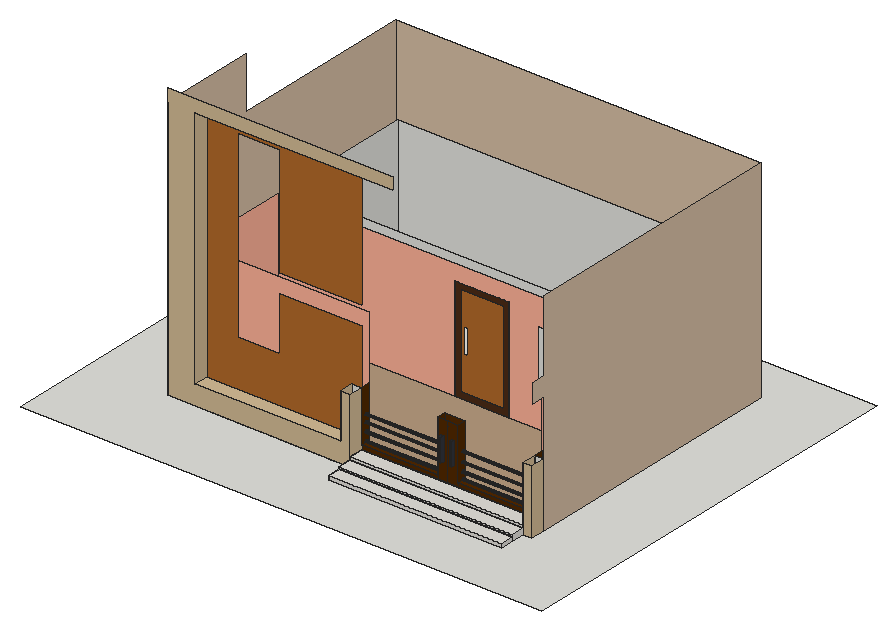
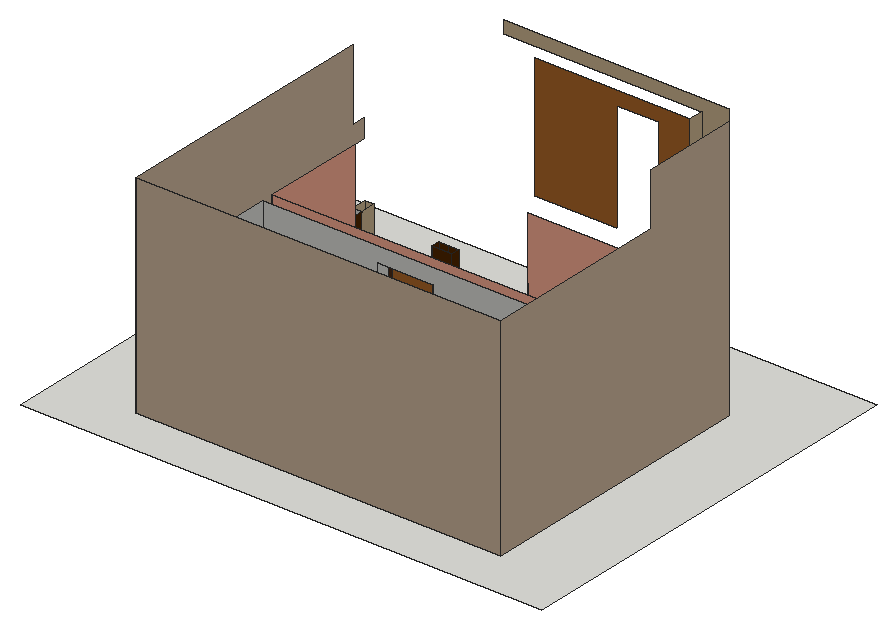
# SketchUp Ruby script. Lengths in inches.
U = 1.inch
M = Sketchup.active_model
def pt(a) = Geom::Point3d.new(a.map { |v| v * U })
def face(e, loops, mat)
  f = e.add_face(loops[0].map { |a| pt(a) })
  loops[1..].each { |l| e.add_face(l.map { |a| pt(a) }).erase! }
  f.material = f.back_material = mat if mat
  f
end
# faces: each face lists its corners as indices into pts; further lists are holes
def faces(e, pts, list, mat = nil) = list.each { |f| face(e, (f[0].is_a?(Array) ? f : [f]).map { |l| l.map { |i| pts[i] } }, mat) }
# xy, xz, yz: faces in a plane at the given z, y or x. An outline is a flat list of corners, or four numbers for a rectangle; further outlines are holes
def ring(l) = l.size == 4 ? [[l[0], l[1]], [l[2], l[1]], [l[2], l[3]], [l[0], l[3]]] : l.each_slice(2).to_a
def flat(e, list, mat, &to3) = list.each { |f| face(e, (f[0].is_a?(Array) ? f : [f]).map { |l| ring(l).map { |u, v| to3.(u, v) } }, mat) }
def xy(e, z, list, mat = nil) = flat(e, list, mat) { |x, y| [x, y, z] }
def xz(e, y, list, mat = nil) = flat(e, list, mat) { |x, z| [x, y, z] }
def yz(e, x, list, mat = nil) = flat(e, list, mat) { |y, z| [x, y, z] }
def lines(e, pts, list) = list.each { |a, b| e.add_line(pt(pts[a]), pt(pts[b])) }
# prism: a flat outline (further loops are holes) pulled along v
def prism(e, loops, v, mat = nil)
  f = face(e, loops, mat); d = Geom::Vector3d.new(v.map { |x| x * U })
  f.pushpull(f.normal.samedirection?(d) ? d.length : -d.length)
end
def box(e, o, s, mat = nil) = prism(e, [[o, [o[0] + s[0], o[1], o[2]], [o[0] + s[0], o[1] + s[1], o[2]], [o[0], o[1] + s[1], o[2]]]], [0, 0, s[2]], mat)
def at(x, y, z, deg = 0) = Geom::Transformation.translation(pt([x, y, z])) * Geom::Transformation.rotation(ORIGIN, Z_AXIS, deg.degrees)
def axes(o, x, y, z) = Geom::Transformation.new([*x, 0, *y, 0, *z, 0, *pt(o).to_a, 1])
def part(name) = M.definitions.add(name)
# library, detail: a bought-in or finely detailed component or shape, given as its bounding box
def library(name, o, s) = part(name).tap { |d| box(d.entities, o, s) }
def detail(e, o, s) = box(e.add_group.entities, o, s)
def put(e, d, t, mat = nil) = e.add_instance(d, t).tap { |i| i.material = mat if mat }
def group(e, t, mat = nil) = e.add_group.tap { |g| g.transformation = t; g.material = mat if mat }.entities
root = M.entities
M.materials.add("[Carpet Pattern Leaf Squares Tan]").color = [181, 154, 125]
M.materials.add("[Color B02]").color = [255, 178, 153]
M.materials.add("[Color C07]").color = [81, 40, 0]
M.materials.add("[Formica Beige]").color = [211, 187, 149]
M.materials.add("[Formica Laminate Dark]").color = [50, 53, 60]
M.materials.add("[Formica Laminate Light]").color = [213, 189, 164]
M.materials.add("[Marble Carrara Gold Floor Tile]").color = [225, 223, 217]
M.materials.add("[Wood Bamboo]").color = [177, 105, 43]
M.materials.add("[Wood Veneer 01]").color = [76, 44, 23]
xy(root,0,[[[0,0,523.75,420.4375],[262.04,59.3,436.45,59.3,436.45,86.05,445.45,86.05,445.45,373.42,79.02,373.42,79.02,86.05,262.04,86.05]],[262.04,59.3,436.45,72.67],[262.04,72.67,436.45,86.05],[79.02,86.05,79.02,373.42,445.45,373.42,445.45,100.8,246.1,100.8,246.1,86.05],[246.1,86.05,262.24,100.8],
  [262.24,86.05,436.45,100.8],[436.45,86.05,445.45,100.8]])
xy(root,3.75,[[262.04,59.3,436.45,72.67]],"[Marble Carrara Gold Floor Tile]")
xy(root,6.125,[[262.04,72.67,436.45,86.05]],"[Marble Carrara Gold Floor Tile]")
xy(root,9,[[266,213.0625,320.78,224.66],[88.02,224.66,436.45,364.42]])
xy(root,9,[[88.02,109.8,436.45,213.0625]],"[Carpet Pattern Leaf Squares Tan]")
xy(root,9,[[262.24,86.05,436.45,100.8]],"[Marble Carrara Gold Floor Tile]")
xy(root,13.11,[[359.13,106.01,436.45,109.8]])
xy(root,13.11,[[262.24,100.8,338.39,109.8],[359.13,100.8,436.45,106.01]],"[Color C07]")
xy(root,19.9,[[106.35,86.05,252.91,100.8]],"[Formica Beige]")
xy(root,27.09,[[342.13,97.98,344.57,100.8],[352.82,97.98,355.26,100.8]],"[Formica Laminate Dark]")
xz(root,59.3,[[262.04,0,436.45,3.75]],"[Marble Carrara Gold Floor Tile]")
xz(root,72.67,[[262.04,0,436.45,3.75]])
xz(root,72.67,[[262.04,3.75,436.45,6.125]],"[Marble Carrara Gold Floor Tile]")
xz(root,86.05,[[262.04,0,262.24,6.125],[262.24,0,436.45,6.125],[262.04,6.125,262.24,64.77]])
xz(root,86.05,[[79.02,0,262.04,0,262.04,64.77,252.91,64.77,252.91,19.9,106.35,19.9,106.35,264.08,305.61,264.08,305.61,276.4375,79.02,276.4375],[436.45,0,445.45,64.77]],"[Formica Beige]")
xz(root,86.05,[[262.24,6.125,436.45,9]],"[Marble Carrara Gold Floor Tile]")
xz(root,97.98,[[342.13,27.09,344.57,49.9],[352.82,27.09,355.26,49.9]],"[Formica Laminate Dark]")
xz(root,100.8,[[246.1,0,262.24,0,262.24,64.77,252.91,64.77,252.91,19.9,246.1,19.9],[262.24,0,338.39,9],[338.39,0,348.76,9],[348.76,0,359.13,9],[359.13,0,436.45,9],
  [436.45,0,445.45,64.77]])
xz(root,100.8,[[262.24,9,338.39,13.11],[[338.39,9,348.76,64.77],[342.13,27.09,344.57,49.9]],[[348.76,9,359.13,64.77],[352.82,27.09,355.26,49.9]],[359.13,9,436.45,13.11]],"[Color C07]")
xz(root,100.8,[[106.35,19.9,252.91,19.9,252.91,64.77,262.24,64.77,262.24,120.54,180.23,120.54,180.23,66.71,137.86,66.71,137.86,250,180.23,250,180.23,139.625,262.24,139.625,262.24,264.08,106.35,264.08]],"[Wood Bamboo]")
xz(root,109.8,[[262.24,9,338.39,13.11],[359.13,9,436.45,13.11]])
xz(root,109.8,[[88.02,9,262.24,129]],"[Color B02]")
xz(root,109.8,[[338.39,9,359.13,64.77]],"[Color C07]")
xz(root,213.0625,[[[88.02,9,266,9,266,113.3,320.78,113.3,320.78,9,436.45,9,436.45,129,88.02,129],[349.875,43.38,418,101.95]]],"[Color B02]")
xz(root,213.0625,[[[271.87,14.87,314.91,107.4375],[275.21,50.38,279.02,74.76]]],"[Wood Bamboo]")
xz(root,213.0625,[[[266,9,320.78,113.3],[271.87,14.87,314.91,107.4375]]],"[Wood Veneer 01]")
xz(root,224.66,[[[88.02,9,88.02,129,436.45,129,436.45,9,320.78,9,320.78,113.3,266,113.3,266,9],[349.875,43.38,418,101.95]]])
xz(root,364.42,[[88.02,9,436.45,129]])
xz(root,373.42,[[79.02,0,445.45,211.625]],"[Formica Laminate Light]")
yz(root,79.02,[[86.05,0,86.05,264.08,184.36,264.08,184.36,211.625,373.42,211.625,373.42,0]],"[Formica Laminate Light]")
yz(root,88.02,[[224.66,9,364.42,129]])
yz(root,88.02,[[109.8,9,213.0625,129]],"[Color B02]")
yz(root,106.35,[[86.05,19.9,100.8,264.08]],"[Formica Beige]")
yz(root,252.91,[[86.05,19.9,100.8,64.77]],"[Formica Beige]")
yz(root,262.04,[[59.3,0,72.67,3.75],[72.67,0,86.05,6.125]],"[Marble Carrara Gold Floor Tile]")
yz(root,262.24,[[86.05,0,100.8,9],[105.68,13.86,105.43,13.9,105.18,14,104.98,14.15,104.82,14.36,104.72,14.6,104.68,14.86,104.72,15.12,104.82,15.36,104.98,15.57,105.18,15.73,105.43,15.83,105.68,15.86,105.94,15.83,106.18,15.73,106.39,15.57,106.55,15.36,106.65,15.12,106.68,14.86,106.65,14.6,106.55,14.36,106.39,14.15,106.18,14,105.94,13.9],[105.68,22.36,105.43,22.4,105.18,22.5,104.98,22.65,104.82,22.86,104.72,23.1,104.68,23.36,104.72,23.62,104.82,23.86,104.98,24.07,105.18,24.23,105.43,24.33,105.68,24.36,105.94,24.33,106.18,24.23,106.39,24.07,106.55,23.86,106.65,23.62,106.68,23.36,106.65,23.1,106.55,22.86,106.39,22.65,106.18,22.5,105.94,22.4],[105.68,30.61,105.43,30.65,105.18,30.75,104.98,30.9,104.82,31.11,104.72,31.35,104.68,31.61,104.72,31.87,104.82,32.11,104.98,32.32,105.18,32.48,105.43,32.58,105.68,32.61,105.94,32.58,106.18,32.48,106.39,32.32,106.55,32.11,106.65,31.87,106.68,31.61,106.65,31.35,106.55,31.11,106.39,30.9,106.18,30.75,105.94,30.65],[105.68,38.11,105.43,38.15,105.18,38.25,104.98,38.4,104.82,38.61,104.72,38.85,104.68,39.11,104.72,39.37,104.82,39.61,104.98,39.82,105.18,39.98,105.43,40.08,105.68,40.11,105.94,40.08,106.18,39.98,106.39,39.82,106.55,39.61,106.65,39.37,106.68,39.11,106.65,38.85,106.55,38.61,106.39,38.4,106.18,38.25,105.94,38.15]])
yz(root,262.24,[[[100.8,13.11,109.8,64.77],[105.68,13.86,105.43,13.9,105.18,14,104.98,14.15,104.82,14.36,104.72,14.6,104.68,14.86,104.72,15.12,104.82,15.36,104.98,15.57,105.18,15.73,105.43,15.83,105.68,15.86,105.94,15.83,106.18,15.73,106.39,15.57,106.55,15.36,106.65,15.12,106.68,14.86,106.65,14.6,106.55,14.36,106.39,14.15,106.18,14,105.94,13.9],[105.68,53.61,105.43,53.65,105.18,53.75,104.98,53.9,104.82,54.11,104.72,54.35,104.68,54.61,104.72,54.87,104.82,55.11,104.98,55.32,105.18,55.48,105.43,55.58,105.68,55.61,105.94,55.58,106.18,55.48,106.39,55.32,106.55,55.11,106.65,54.87,106.68,54.61,106.65,54.35,106.55,54.11,106.39,53.9,106.18,53.75,105.94,53.65],[105.68,22.36,105.43,22.4,105.18,22.5,104.98,22.65,104.82,22.86,104.72,23.1,104.68,23.36,104.72,23.62,104.82,23.86,104.98,24.07,105.18,24.23,105.43,24.33,105.68,24.36,105.94,24.33,106.18,24.23,106.39,24.07,106.55,23.86,106.65,23.62,106.68,23.36,106.65,23.1,106.55,22.86,106.39,22.65,106.18,22.5,105.94,22.4],[105.68,45.42,105.43,45.46,105.18,45.56,104.98,45.72,104.82,45.92,104.72,46.17,104.68,46.42,104.72,46.68,104.82,46.92,104.98,47.13,105.18,47.29,105.43,47.39,105.68,47.42,105.94,47.39,106.18,47.29,106.39,47.13,106.55,46.92,106.65,46.68,106.68,46.42,106.65,46.17,106.55,45.92,106.39,45.72,106.18,45.56,105.94,45.46],[105.68,30.61,105.43,30.65,105.18,30.75,104.98,30.9,104.82,31.11,104.72,31.35,104.68,31.61,104.72,31.87,104.82,32.11,104.98,32.32,105.18,32.48,105.43,32.58,105.68,32.61,105.94,32.58,106.18,32.48,106.39,32.32,106.55,32.11,106.65,31.87,106.68,31.61,106.65,31.35,106.55,31.11,106.39,30.9,106.18,30.75,105.94,30.65],[105.68,38.11,105.43,38.15,105.18,38.25,104.98,38.4,104.82,38.61,104.72,38.85,104.68,39.11,104.72,39.37,104.82,39.61,104.98,39.82,105.18,39.98,105.43,40.08,105.68,40.11,105.94,40.08,106.18,39.98,106.39,39.82,106.55,39.61,106.65,39.37,106.68,39.11,106.65,38.85,106.55,38.61,106.39,38.4,106.18,38.25,105.94,38.15],[105.68,60.05,105.43,60.08,105.18,60.18,104.98,60.34,104.82,60.55,104.72,60.79,104.68,61.05,104.72,61.31,104.82,61.55,104.98,61.76,105.18,61.92,105.43,62.02,105.68,62.05,105.94,62.02,106.18,61.92,106.39,61.76,106.55,61.55,106.65,61.31,106.68,61.05,106.65,60.79,106.55,60.55,106.39,60.34,106.18,60.18,105.94,60.08]]],"[Color C07]")
yz(root,262.24,[[86.05,9,100.8,64.77]],"[Formica Beige]")
yz(root,266,[[213.0625,9,224.66,113.3]])
yz(root,320.78,[[213.0625,9,224.66,113.3]])
yz(root,338.39,[[[100.8,13.11,109.8,64.77],[105.68,60.05,105.94,60.08,106.18,60.18,106.39,60.34,106.55,60.55,106.65,60.79,106.68,61.05,106.65,61.31,106.55,61.55,106.39,61.76,106.18,61.92,105.94,62.02,105.68,62.05,105.43,62.02,105.18,61.92,104.98,61.76,104.82,61.55,104.72,61.31,104.68,61.05,104.72,60.79,104.82,60.55,104.98,60.34,105.18,60.18,105.43,60.08],[105.68,53.61,105.94,53.65,106.18,53.75,106.39,53.9,106.55,54.11,106.65,54.35,106.68,54.61,106.65,54.87,106.55,55.11,106.39,55.32,106.18,55.48,105.94,55.58,105.68,55.61,105.43,55.58,105.18,55.48,104.98,55.32,104.82,55.11,104.72,54.87,104.68,54.61,104.72,54.35,104.82,54.11,104.98,53.9,105.18,53.75,105.43,53.65],[105.68,45.42,105.94,45.46,106.18,45.56,106.39,45.72,106.55,45.92,106.65,46.17,106.68,46.42,106.65,46.68,106.55,46.92,106.39,47.13,106.18,47.29,105.94,47.39,105.68,47.42,105.43,47.39,105.18,47.29,104.98,47.13,104.82,46.92,104.72,46.68,104.68,46.42,104.72,46.17,104.82,45.92,104.98,45.72,105.18,45.56,105.43,45.46],[105.68,38.11,105.94,38.15,106.18,38.25,106.39,38.4,106.55,38.61,106.65,38.85,106.68,39.11,106.65,39.37,106.55,39.61,106.39,39.82,106.18,39.98,105.94,40.08,105.68,40.11,105.43,40.08,105.18,39.98,104.98,39.82,104.82,39.61,104.72,39.37,104.68,39.11,104.72,38.85,104.82,38.61,104.98,38.4,105.18,38.25,105.43,38.15],[105.68,30.61,105.94,30.65,106.18,30.75,106.39,30.9,106.55,31.11,106.65,31.35,106.68,31.61,106.65,31.87,106.55,32.11,106.39,32.32,106.18,32.48,105.94,32.58,105.68,32.61,105.43,32.58,105.18,32.48,104.98,32.32,104.82,32.11,104.72,31.87,104.68,31.61,104.72,31.35,104.82,31.11,104.98,30.9,105.18,30.75,105.43,30.65],[105.68,22.36,105.94,22.4,106.18,22.5,106.39,22.65,106.55,22.86,106.65,23.1,106.68,23.36,106.65,23.62,106.55,23.86,106.39,24.07,106.18,24.23,105.94,24.33,105.68,24.36,105.43,24.33,105.18,24.23,104.98,24.07,104.82,23.86,104.72,23.62,104.68,23.36,104.72,23.1,104.82,22.86,104.98,22.65,105.18,22.5,105.43,22.4],[105.68,13.86,105.94,13.9,106.18,14,106.39,14.15,106.55,14.36,106.65,14.6,106.68,14.86,106.65,15.12,106.55,15.36,106.39,15.57,106.18,15.73,105.94,15.83,105.68,15.86,105.43,15.83,105.18,15.73,104.98,15.57,104.82,15.36,104.72,15.12,104.68,14.86,104.72,14.6,104.82,14.36,104.98,14.15,105.18,14,105.43,13.9]]],"[Color C07]")
yz(root,342.13,[[97.98,27.09,100.8,49.9]],"[Formica Laminate Dark]")
yz(root,344.57,[[97.98,27.09,100.8,49.9]],"[Formica Laminate Dark]")
yz(root,352.82,[[97.98,27.09,100.8,49.9]],"[Formica Laminate Dark]")
yz(root,355.26,[[97.98,27.09,100.8,49.9]],"[Formica Laminate Dark]")
yz(root,359.13,[[[100.8,13.11,109.8,64.77],[106.01,60.17,105.75,60.2,105.51,60.3,105.3,60.46,105.14,60.67,105.04,60.91,105.01,61.17,105.04,61.43,105.14,61.67,105.3,61.875,105.51,62.03,105.75,62.13,106.01,62.17,106.27,62.13,106.51,62.03,106.72,61.875,106.875,61.67,106.98,61.43,107.01,61.17,106.98,60.91,106.875,60.67,106.72,60.46,106.51,60.3,106.27,60.2],[106.01,53.17,105.75,53.2,105.51,53.3,105.3,53.46,105.14,53.67,105.04,53.91,105.01,54.17,105.04,54.43,105.14,54.67,105.3,54.875,105.51,55.03,105.75,55.13,106.01,55.17,106.27,55.13,106.51,55.03,106.72,54.875,106.875,54.67,106.98,54.43,107.01,54.17,106.98,53.91,106.875,53.67,106.72,53.46,106.51,53.3,106.27,53.2],[106.01,46.23,105.75,46.26,105.51,46.36,105.3,46.52,105.14,46.73,105.04,46.97,105.01,47.23,105.04,47.49,105.14,47.73,105.3,47.9375,105.51,48.1,105.75,48.2,106.01,48.23,106.27,48.2,106.51,48.1,106.72,47.9375,106.875,47.73,106.98,47.49,107.01,47.23,106.98,46.97,106.875,46.73,106.72,46.52,106.51,46.36,106.27,46.26],[106.01,38.36,105.75,38.39,105.51,38.49,105.3,38.65,105.14,38.86,105.04,39.1,105.01,39.36,105.04,39.61,105.14,39.86,105.3,40.0625,105.51,40.22,105.75,40.32,106.01,40.36,106.27,40.32,106.51,40.22,106.72,40.0625,106.875,39.86,106.98,39.61,107.01,39.36,106.98,39.1,106.875,38.86,106.72,38.65,106.51,38.49,106.27,38.39],[106.01,28.73,105.75,28.76,105.51,28.86,105.3,29.02,105.14,29.23,105.04,29.47,105.01,29.73,105.04,29.99,105.14,30.23,105.3,30.4375,105.51,30.6,105.75,30.7,106.01,30.73,106.27,30.7,106.51,30.6,106.72,30.4375,106.875,30.23,106.98,29.99,107.01,29.73,106.98,29.47,106.875,29.23,106.72,29.02,106.51,28.86,106.27,28.76],[106.01,19.98,105.75,20.01,105.51,20.11,105.3,20.27,105.14,20.48,105.04,20.72,105.01,20.98,105.04,21.24,105.14,21.48,105.3,21.6875,105.51,21.85,105.75,21.95,106.01,21.98,106.27,21.95,106.51,21.85,106.72,21.6875,106.875,21.48,106.98,21.24,107.01,20.98,106.98,20.72,106.875,20.48,106.72,20.27,106.51,20.11,106.27,20.01],[106.01,13.11,105.75,13.14,105.51,13.24,105.3,13.4,105.14,13.61,105.04,13.85,105.01,14.11,105.04,14.36,105.14,14.61,105.3,14.8125,105.51,14.97,105.75,15.07,106.01,15.11,106.27,15.07,106.51,14.97,106.72,14.8125,106.875,14.61,106.98,14.36,107.01,14.11,106.98,13.85,106.875,13.61,106.72,13.4,106.51,13.24,106.27,13.14]]],"[Color C07]")
yz(root,436.45,[[86.05,0,100.8,9],[224.66,9,364.42,129],[106.01,13.11,106.27,13.14,106.51,13.24,106.72,13.4,106.875,13.61,106.98,13.85,107.01,14.11,106.98,14.36,106.875,14.61,106.72,14.8125,106.51,14.97,106.27,15.07,106.01,15.11,105.75,15.07,105.51,14.97,105.3,14.8125,105.14,14.61,105.04,14.36,105.01,14.11,105.04,13.85,105.14,13.61,105.3,13.4,105.51,13.24,105.75,13.14],[106.01,19.98,106.27,20.01,106.51,20.11,106.72,20.27,106.875,20.48,106.98,20.72,107.01,20.98,106.98,21.24,106.875,21.48,106.72,21.6875,106.51,21.85,106.27,21.95,106.01,21.98,105.75,21.95,105.51,21.85,105.3,21.6875,105.14,21.48,105.04,21.24,105.01,20.98,105.04,20.72,105.14,20.48,105.3,20.27,105.51,20.11,105.75,20.01],[106.01,28.73,106.27,28.76,106.51,28.86,106.72,29.02,106.875,29.23,106.98,29.47,107.01,29.73,106.98,29.99,106.875,30.23,106.72,30.4375,106.51,30.6,106.27,30.7,106.01,30.73,105.75,30.7,105.51,30.6,105.3,30.4375,105.14,30.23,105.04,29.99,105.01,29.73,105.04,29.47,105.14,29.23,105.3,29.02,105.51,28.86,105.75,28.76],
  [106.01,38.36,106.27,38.39,106.51,38.49,106.72,38.65,106.875,38.86,106.98,39.1,107.01,39.36,106.98,39.61,106.875,39.86,106.72,40.0625,106.51,40.22,106.27,40.32,106.01,40.36,105.75,40.32,105.51,40.22,105.3,40.0625,105.14,39.86,105.04,39.61,105.01,39.36,105.04,39.1,105.14,38.86,105.3,38.65,105.51,38.49,105.75,38.39]])
yz(root,436.45,[[109.8,9,213.0625,129]],"[Color B02]")
yz(root,436.45,[[[100.8,13.11,109.8,64.77],[106.01,13.11,106.27,13.14,106.51,13.24,106.72,13.4,106.875,13.61,106.98,13.85,107.01,14.11,106.98,14.36,106.875,14.61,106.72,14.8125,106.51,14.97,106.27,15.07,106.01,15.11,105.75,15.07,105.51,14.97,105.3,14.8125,105.14,14.61,105.04,14.36,105.01,14.11,105.04,13.85,105.14,13.61,105.3,13.4,105.51,13.24,105.75,13.14],[106.01,53.17,106.27,53.2,106.51,53.3,106.72,53.46,106.875,53.67,106.98,53.91,107.01,54.17,106.98,54.43,106.875,54.67,106.72,54.875,106.51,55.03,106.27,55.13,106.01,55.17,105.75,55.13,105.51,55.03,105.3,54.875,105.14,54.67,105.04,54.43,105.01,54.17,105.04,53.91,105.14,53.67,105.3,53.46,105.51,53.3,105.75,53.2],[106.01,19.98,106.27,20.01,106.51,20.11,106.72,20.27,106.875,20.48,106.98,20.72,107.01,20.98,106.98,21.24,106.875,21.48,106.72,21.6875,106.51,21.85,106.27,21.95,106.01,21.98,105.75,21.95,105.51,21.85,105.3,21.6875,105.14,21.48,105.04,21.24,105.01,20.98,105.04,20.72,105.14,20.48,105.3,20.27,105.51,20.11,105.75,20.01],[106.01,46.23,106.27,46.26,106.51,46.36,106.72,46.52,106.875,46.73,106.98,46.97,107.01,47.23,106.98,47.49,106.875,47.73,106.72,47.9375,106.51,48.1,106.27,48.2,106.01,48.23,105.75,48.2,105.51,48.1,105.3,47.9375,105.14,47.73,105.04,47.49,105.01,47.23,105.04,46.97,105.14,46.73,105.3,46.52,105.51,46.36,105.75,46.26],[106.01,28.73,106.27,28.76,106.51,28.86,106.72,29.02,106.875,29.23,106.98,29.47,107.01,29.73,106.98,29.99,106.875,30.23,106.72,30.4375,106.51,30.6,106.27,30.7,106.01,30.73,105.75,30.7,105.51,30.6,105.3,30.4375,105.14,30.23,105.04,29.99,105.01,29.73,105.04,29.47,105.14,29.23,105.3,29.02,105.51,28.86,105.75,28.76],[106.01,38.36,106.27,38.39,106.51,38.49,106.72,38.65,106.875,38.86,106.98,39.1,107.01,39.36,106.98,39.61,106.875,39.86,106.72,40.0625,106.51,40.22,106.27,40.32,106.01,40.36,105.75,40.32,105.51,40.22,105.3,40.0625,105.14,39.86,105.04,39.61,105.01,39.36,105.04,39.1,105.14,38.86,105.3,38.65,105.51,38.49,105.75,38.39],[106.01,60.17,106.27,60.2,106.51,60.3,106.72,60.46,106.875,60.67,106.98,60.91,107.01,61.17,106.98,61.43,106.875,61.67,106.72,61.875,106.51,62.03,106.27,62.13,106.01,62.17,105.75,62.13,105.51,62.03,105.3,61.875,105.14,61.67,105.04,61.43,105.01,61.17,105.04,60.91,105.14,60.67,105.3,60.46,105.51,60.3,105.75,60.2]]],"[Color C07]")
yz(root,436.45,[[86.05,9,100.8,64.77]],"[Formica Beige]")
yz(root,436.45,[[59.3,0,72.67,3.75],[72.67,0,86.05,6.125]],"[Marble Carrara Gold Floor Tile]")
yz(root,445.45,[[86.05,0,100.8,64.77]],"[Formica Beige]")
yz(root,445.45,[[100.8,0,373.42,0,373.42,211.625,100.8,211.625,100.8,139.625,86.42,139.625,86.42,120.54,100.8,120.54]],"[Formica Laminate Light]")
p = [[436.45,105.75,13.14],[436.45,105.51,13.24],[359.13,105.51,13.24],[359.13,105.75,13.14],[436.45,106.01,13.11],[359.13,106.01,13.11],
  [436.45,106.27,13.14],[359.13,106.27,13.14],[436.45,106.51,13.24],[359.13,106.51,13.24],[436.45,105.3,13.4],[359.13,105.3,13.4],
  [436.45,106.72,13.4],[359.13,106.72,13.4],[436.45,105.14,13.61],[359.13,105.14,13.61],[436.45,106.875,13.61],[359.13,106.875,13.61],
  [436.45,105.04,13.85],[359.13,105.04,13.85],[436.45,106.98,13.85],[359.13,106.98,13.85],[436.45,105.01,14.11],[359.13,105.01,14.11],
  [436.45,107.01,14.11],[359.13,107.01,14.11],[262.24,105.18,14],[262.24,105.43,13.9],[338.39,105.43,13.9],[338.39,105.18,14],
  [262.24,105.68,13.86],[338.39,105.68,13.86],[262.24,105.94,13.9],[338.39,105.94,13.9],[262.24,106.18,14],[338.39,106.18,14],
  [262.24,104.98,14.15],[338.39,104.98,14.15],[262.24,106.39,14.15],[338.39,106.39,14.15],[436.45,105.04,14.36],[359.13,105.04,14.36],
  [436.45,106.98,14.36],[359.13,106.98,14.36],[262.24,104.82,14.36],[338.39,104.82,14.36],[262.24,106.55,14.36],[338.39,106.55,14.36],
  [262.24,104.72,14.6],[338.39,104.72,14.6],[436.45,105.14,14.61],[359.13,105.14,14.61],[262.24,106.65,14.6],[338.39,106.65,14.6],
  [436.45,106.875,14.61],[359.13,106.875,14.61],[262.24,104.68,14.86],[338.39,104.68,14.86],[436.45,105.3,14.8125],[359.13,105.3,14.8125],
  [262.24,106.68,14.86],[338.39,106.68,14.86],[436.45,106.72,14.8125],[359.13,106.72,14.8125],[436.45,105.51,14.97],[359.13,105.51,14.97],
  [436.45,106.51,14.97],[359.13,106.51,14.97],[262.24,104.72,15.12],[338.39,104.72,15.12],[262.24,106.65,15.12],[338.39,106.65,15.12],
  [436.45,105.75,15.07],[359.13,105.75,15.07],[436.45,106.27,15.07],[359.13,106.27,15.07],[262.24,104.82,15.36],[338.39,104.82,15.36],
  [436.45,106.01,15.11],[359.13,106.01,15.11],[262.24,106.55,15.36],[338.39,106.55,15.36],[262.24,104.98,15.57],[338.39,104.98,15.57],
  [262.24,106.39,15.57],[338.39,106.39,15.57],[262.24,105.18,15.73],[338.39,105.18,15.73],[262.24,106.18,15.73],[338.39,106.18,15.73],
  [262.24,105.43,15.83],[338.39,105.43,15.83],[262.24,105.94,15.83],[338.39,105.94,15.83],[262.24,105.68,15.86],[338.39,105.68,15.86],
  [436.45,105.75,20.01],[436.45,105.51,20.11],[359.13,105.51,20.11],[359.13,105.75,20.01],[436.45,106.01,19.98],[359.13,106.01,19.98],
  [436.45,106.27,20.01],[359.13,106.27,20.01],[436.45,106.51,20.11],[359.13,106.51,20.11],[436.45,105.3,20.27],[359.13,105.3,20.27],
  [436.45,106.72,20.27],[359.13,106.72,20.27],[436.45,105.14,20.48],[359.13,105.14,20.48],[436.45,106.875,20.48],[359.13,106.875,20.48],
  [436.45,105.04,20.72],[359.13,105.04,20.72],[436.45,106.98,20.72],[359.13,106.98,20.72],[436.45,105.01,20.98],[359.13,105.01,20.98],
  [436.45,107.01,20.98],[359.13,107.01,20.98],[436.45,105.04,21.24],[359.13,105.04,21.24],[436.45,106.98,21.24],[359.13,106.98,21.24],
  [436.45,105.14,21.48],[359.13,105.14,21.48],[436.45,106.875,21.48],[359.13,106.875,21.48],[436.45,105.3,21.6875],[359.13,105.3,21.6875],
  [436.45,106.72,21.6875],[359.13,106.72,21.6875],[436.45,105.51,21.85],[359.13,105.51,21.85],[436.45,106.51,21.85],[359.13,106.51,21.85],
  [436.45,105.75,21.95],[359.13,105.75,21.95],[436.45,106.27,21.95],[359.13,106.27,21.95],[436.45,106.01,21.98],[359.13,106.01,21.98],
  [262.24,105.18,22.5],[262.24,105.43,22.4],[338.39,105.43,22.4],[338.39,105.18,22.5],[262.24,105.68,22.36],[338.39,105.68,22.36],
  [262.24,105.94,22.4],[338.39,105.94,22.4],[262.24,106.18,22.5],[338.39,106.18,22.5],[262.24,104.98,22.65],[338.39,104.98,22.65],
  [262.24,106.39,22.65],[338.39,106.39,22.65],[262.24,104.82,22.86],[338.39,104.82,22.86],[262.24,106.55,22.86],[338.39,106.55,22.86],
  [262.24,104.72,23.1],[338.39,104.72,23.1],[262.24,106.65,23.1],[338.39,106.65,23.1],[262.24,104.68,23.36],[338.39,104.68,23.36],
  [262.24,106.68,23.36],[338.39,106.68,23.36],[262.24,104.72,23.62],[338.39,104.72,23.62],[262.24,106.65,23.62],[338.39,106.65,23.62],
  [262.24,104.82,23.86],[338.39,104.82,23.86],[262.24,106.55,23.86],[338.39,106.55,23.86],[262.24,104.98,24.07],[338.39,104.98,24.07],
  [262.24,106.39,24.07],[338.39,106.39,24.07],[262.24,105.18,24.23],[338.39,105.18,24.23],[262.24,106.18,24.23],[338.39,106.18,24.23],
  [262.24,105.43,24.33],[338.39,105.43,24.33],[262.24,105.94,24.33],[338.39,105.94,24.33],[262.24,105.68,24.36],[338.39,105.68,24.36],
  [436.45,106.01,28.73],[436.45,105.75,28.76],[359.13,105.75,28.76],[359.13,106.01,28.73],[436.45,106.27,28.76],[359.13,106.27,28.76],
  [436.45,105.51,28.86],[359.13,105.51,28.86],[436.45,106.51,28.86],[359.13,106.51,28.86],[436.45,105.3,29.02],[359.13,105.3,29.02],
  [436.45,106.72,29.02],[359.13,106.72,29.02],[436.45,105.14,29.23],[359.13,105.14,29.23],[436.45,106.875,29.23],[359.13,106.875,29.23],
  [436.45,105.04,29.47],[359.13,105.04,29.47],[436.45,106.98,29.47],[359.13,106.98,29.47],[436.45,105.01,29.73],[359.13,105.01,29.73],
  [436.45,107.01,29.73],[359.13,107.01,29.73],[436.45,105.04,29.99],[359.13,105.04,29.99],[436.45,106.98,29.99],[359.13,106.98,29.99],
  [436.45,105.14,30.23],[359.13,105.14,30.23],[436.45,106.875,30.23],[359.13,106.875,30.23],[436.45,105.3,30.4375],[359.13,105.3,30.4375],
  [436.45,106.72,30.4375],[359.13,106.72,30.4375],[436.45,105.51,30.6],[359.13,105.51,30.6],[436.45,106.51,30.6],[359.13,106.51,30.6],
  [262.24,105.18,30.75],[262.24,105.43,30.65],[338.39,105.43,30.65],[338.39,105.18,30.75],[262.24,105.68,30.61],[338.39,105.68,30.61],
  [436.45,105.75,30.7],[359.13,105.75,30.7],[262.24,105.94,30.65],[338.39,105.94,30.65],[262.24,106.18,30.75],[338.39,106.18,30.75],
  [436.45,106.27,30.7],[359.13,106.27,30.7],[262.24,104.98,30.9],[338.39,104.98,30.9],[436.45,106.01,30.73],[359.13,106.01,30.73],
  [262.24,106.39,30.9],[338.39,106.39,30.9],[262.24,104.82,31.11],[338.39,104.82,31.11],[262.24,106.55,31.11],[338.39,106.55,31.11],
  [262.24,104.72,31.35],[338.39,104.72,31.35],[262.24,106.65,31.35],[338.39,106.65,31.35],[262.24,104.68,31.61],[338.39,104.68,31.61],
  [262.24,106.68,31.61],[338.39,106.68,31.61],[262.24,104.72,31.87],[338.39,104.72,31.87],[262.24,106.65,31.87],[338.39,106.65,31.87],
  [262.24,104.82,32.11],[338.39,104.82,32.11],[262.24,106.55,32.11],[338.39,106.55,32.11],[262.24,104.98,32.32],[338.39,104.98,32.32],
  [262.24,106.39,32.32],[338.39,106.39,32.32],[262.24,105.18,32.48],[338.39,105.18,32.48],[262.24,106.18,32.48],[338.39,106.18,32.48],
  [262.24,105.43,32.58],[338.39,105.43,32.58],[262.24,105.94,32.58],[338.39,105.94,32.58],[262.24,105.68,32.61],[338.39,105.68,32.61],
  [262.24,105.18,38.25],[262.24,105.43,38.15],[338.39,105.43,38.15],[338.39,105.18,38.25],[262.24,105.68,38.11],[338.39,105.68,38.11],
  [262.24,105.94,38.15],[338.39,105.94,38.15],[262.24,106.18,38.25],[338.39,106.18,38.25],[262.24,104.98,38.4],[338.39,104.98,38.4],
  [262.24,106.39,38.4],[338.39,106.39,38.4],[262.24,104.82,38.61],[338.39,104.82,38.61],[436.45,105.75,38.39],[436.45,105.51,38.49],
  [359.13,105.51,38.49],[359.13,105.75,38.39],[436.45,106.01,38.36],[359.13,106.01,38.36],[436.45,106.27,38.39],[359.13,106.27,38.39],
  [436.45,106.51,38.49],[359.13,106.51,38.49],[262.24,106.55,38.61],[338.39,106.55,38.61],[436.45,105.3,38.65],[359.13,105.3,38.65],
  [436.45,106.72,38.65],[359.13,106.72,38.65],[262.24,104.72,38.85],[338.39,104.72,38.85],[436.45,105.14,38.86],[359.13,105.14,38.86],
  [262.24,106.65,38.85],[338.39,106.65,38.85],[436.45,106.875,38.86],[359.13,106.875,38.86],[262.24,104.68,39.11],[338.39,104.68,39.11],
  [436.45,105.04,39.1],[359.13,105.04,39.1],[262.24,106.68,39.11],[338.39,106.68,39.11],[436.45,106.98,39.1],[359.13,106.98,39.1],
  [262.24,104.72,39.37],[338.39,104.72,39.37],[436.45,105.01,39.36],[359.13,105.01,39.36],[262.24,106.65,39.37],[338.39,106.65,39.37],
  [436.45,107.01,39.36],[359.13,107.01,39.36],[262.24,104.82,39.61],[338.39,104.82,39.61],[436.45,105.04,39.61],[359.13,105.04,39.61],
  [262.24,106.55,39.61],[338.39,106.55,39.61],[436.45,106.98,39.61],[359.13,106.98,39.61],[262.24,104.98,39.82],[338.39,104.98,39.82],
  [436.45,105.14,39.86],[359.13,105.14,39.86],[262.24,106.39,39.82],[338.39,106.39,39.82],[436.45,106.875,39.86],[359.13,106.875,39.86],
  [262.24,105.18,39.98],[338.39,105.18,39.98],[262.24,106.18,39.98],[338.39,106.18,39.98],[436.45,105.3,40.0625],[359.13,105.3,40.0625],
  [436.45,106.72,40.0625],[359.13,106.72,40.0625],[262.24,105.43,40.08],[338.39,105.43,40.08],[262.24,105.94,40.08],[338.39,105.94,40.08],
  [436.45,105.51,40.22],[359.13,105.51,40.22],[262.24,105.68,40.11],[338.39,105.68,40.11],[436.45,106.51,40.22],[359.13,106.51,40.22],
  [436.45,105.75,40.32],[359.13,105.75,40.32],[436.45,106.27,40.32],[359.13,106.27,40.32],[436.45,106.01,40.36],[359.13,106.01,40.36]]
faces(root,p,[[0,1,2,3],[4,0,3,5],[6,4,5,7],[8,6,7,9],[1,10,11,2],[12,8,9,13],[10,14,15,11],[16,12,13,17],
  [14,18,19,15],[20,16,17,21],[18,22,23,19],[24,20,21,25],[26,27,28,29],[27,30,31,28],[30,32,33,31],[32,34,35,33],
  [36,26,29,37],[34,38,39,35],[22,40,41,23],[42,24,25,43],[44,36,37,45],[38,46,47,39],[48,44,45,49],[40,50,51,41],
  [46,52,53,47],[54,42,43,55],[56,48,49,57],[50,58,59,51],[52,60,61,53],[62,54,55,63],[58,64,65,59],[66,62,63,67],
  [68,56,57,69],[60,70,71,61],[64,72,73,65],[74,66,67,75],[76,68,69,77],[72,78,79,73],[78,74,75,79],[70,80,81,71],
  [82,76,77,83],[80,84,85,81],[86,82,83,87],[84,88,89,85],[90,86,87,91],[88,92,93,89],[94,90,91,95],[92,94,95,93],
  [96,97,98,99],[100,96,99,101],[102,100,101,103],[104,102,103,105],[97,106,107,98],[108,104,105,109],[106,110,111,107],[112,108,109,113],
  [110,114,115,111],[116,112,113,117],[114,118,119,115],[120,116,117,121],[118,122,123,119],[124,120,121,125],[122,126,127,123],[128,124,125,129],
  [126,130,131,127],[132,128,129,133],[130,134,135,131],[136,132,133,137],[134,138,139,135],[140,136,137,141],[138,142,143,139],[142,140,141,143],
  [144,145,146,147],[145,148,149,146],[148,150,151,149],[150,152,153,151],[154,144,147,155],[152,156,157,153],[158,154,155,159],[156,160,161,157],
  [162,158,159,163],[160,164,165,161],[166,162,163,167],[164,168,169,165],[170,166,167,171],[168,172,173,169],[174,170,171,175],[172,176,177,173],
  [178,174,175,179],[176,180,181,177],[182,178,179,183],[180,184,185,181],[186,182,183,187],[184,188,189,185],[190,186,187,191],[188,190,191,189],
  [192,193,194,195],[196,192,195,197],[193,198,199,194],[200,196,197,201],[198,202,203,199],[204,200,201,205],[202,206,207,203],[208,204,205,209],
  [206,210,211,207],[212,208,209,213],[210,214,215,211],[216,212,213,217],[214,218,219,215],[220,216,217,221],[218,222,223,219],[224,220,221,225],
  [222,226,227,223],[228,224,225,229],[226,230,231,227],[232,228,229,233],[234,235,236,237],[235,238,239,236],[230,240,241,231],[238,242,243,239],
  [242,244,245,243],[246,232,233,247],[248,234,237,249],[240,250,251,241],[250,246,247,251],[244,252,253,245],[254,248,249,255],[252,256,257,253],
  [258,254,255,259],[256,260,261,257],[262,258,259,263],[260,264,265,261],[266,262,263,267],[264,268,269,265],[270,266,267,271],[268,272,273,269],
  [274,270,271,275],[272,276,277,273],[278,274,275,279],[276,280,281,277],[282,278,279,283],[280,284,285,281],[286,282,283,287],[284,286,287,285],
  [288,289,290,291],[289,292,293,290],[292,294,295,293],[294,296,297,295],[298,288,291,299],[296,300,301,297],[302,298,299,303],[304,305,306,307],
  [308,304,307,309],[310,308,309,311],[312,310,311,313],[300,314,315,301],[305,316,317,306],[318,312,313,319],[320,302,303,321],[316,322,323,317],
  [314,324,325,315],[326,318,319,327],[328,320,321,329],[322,330,331,323],[324,332,333,325],[334,326,327,335],[336,328,329,337],[330,338,339,331],
  [332,340,341,333],[342,334,335,343],[344,336,337,345],[338,346,347,339],[340,348,349,341],[350,342,343,351],[352,344,345,353],[346,354,355,347],
  [348,356,357,349],[358,350,351,359],[360,352,353,361],[356,362,363,357],[354,364,365,355],[366,358,359,367],[368,360,361,369],[362,370,371,363],
  [364,372,373,365],[374,368,369,375],[370,374,375,371],[376,366,367,377],[372,378,379,373],[380,376,377,381],[378,382,383,379],[382,380,381,383]],"[Color C07]")
